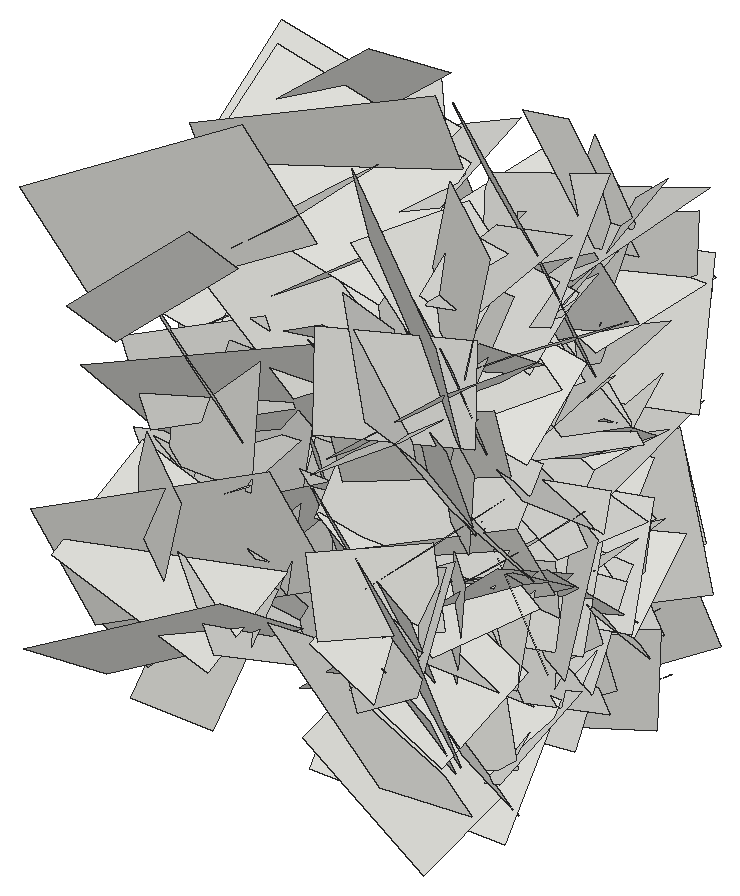
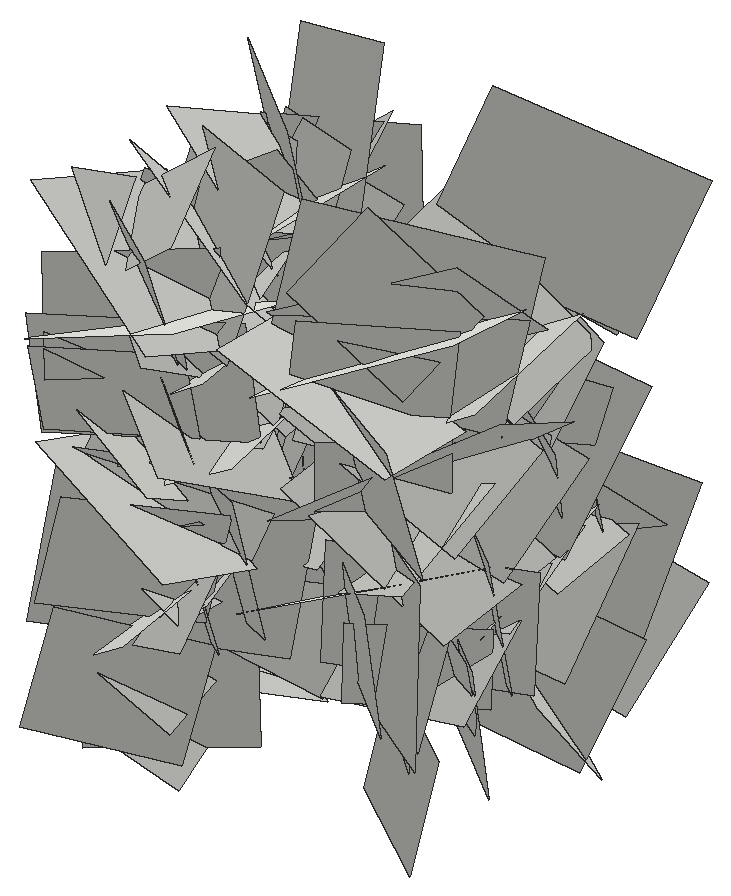
# SketchUp Ruby script. Lengths in inches.
U = 1.inch
M = Sketchup.active_model
def pt(a) = Geom::Point3d.new(a.map { |v| v * U })
def face(e, loops, mat)
  f = e.add_face(loops[0].map { |a| pt(a) })
  loops[1..].each { |l| e.add_face(l.map { |a| pt(a) }).erase! }
  f.material = f.back_material = mat if mat
  f
end
# faces: each face lists its corners as indices into pts; further lists are holes
def faces(e, pts, list, mat = nil) = list.each { |f| face(e, (f[0].is_a?(Array) ? f : [f]).map { |l| l.map { |i| pts[i] } }, mat) }
# xy, xz, yz: faces in a plane at the given z, y or x. An outline is a flat list of corners, or four numbers for a rectangle; further outlines are holes
def ring(l) = l.size == 4 ? [[l[0], l[1]], [l[2], l[1]], [l[2], l[3]], [l[0], l[3]]] : l.each_slice(2).to_a
def flat(e, list, mat, &to3) = list.each { |f| face(e, (f[0].is_a?(Array) ? f : [f]).map { |l| ring(l).map { |u, v| to3.(u, v) } }, mat) }
def xy(e, z, list, mat = nil) = flat(e, list, mat) { |x, y| [x, y, z] }
def xz(e, y, list, mat = nil) = flat(e, list, mat) { |x, z| [x, y, z] }
def yz(e, x, list, mat = nil) = flat(e, list, mat) { |y, z| [x, y, z] }
def lines(e, pts, list) = list.each { |a, b| e.add_line(pt(pts[a]), pt(pts[b])) }
# prism: a flat outline (further loops are holes) pulled along v
def prism(e, loops, v, mat = nil)
  f = face(e, loops, mat); d = Geom::Vector3d.new(v.map { |x| x * U })
  f.pushpull(f.normal.samedirection?(d) ? d.length : -d.length)
end
def box(e, o, s, mat = nil) = prism(e, [[o, [o[0] + s[0], o[1], o[2]], [o[0] + s[0], o[1] + s[1], o[2]], [o[0], o[1] + s[1], o[2]]]], [0, 0, s[2]], mat)
def at(x, y, z, deg = 0) = Geom::Transformation.translation(pt([x, y, z])) * Geom::Transformation.rotation(ORIGIN, Z_AXIS, deg.degrees)
def axes(o, x, y, z) = Geom::Transformation.new([*x, 0, *y, 0, *z, 0, *pt(o).to_a, 1])
def part(name) = M.definitions.add(name)
# library, detail: a bought-in or finely detailed component or shape, given as its bounding box
def library(name, o, s) = part(name).tap { |d| box(d.entities, o, s) }
def detail(e, o, s) = box(e.add_group.entities, o, s)
def put(e, d, t, mat = nil) = e.add_instance(d, t).tap { |i| i.material = mat if mat }
def group(e, t, mat = nil) = e.add_group.tap { |g| g.transformation = t; g.material = mat if mat }.entities
root = M.entities
c1 = part("Component\#6")
p = [[0.01,0,0],[0,3.24,4.54],[4.32,3.24,4.54],[4.33,0,0]]
faces(c1.entities,p,[[0,1,2,3]])
put(root,c1,axes([14.53,152.65,32.7],[-0.31384,1.21799,0.62272],[-0.13011,0.61092,-1.25326],[1.44417,0.31973,0.02242]))
put(root,c1,axes([14.53,149.65,34.23],[-0.2234,-0.54463,1.08834],[-0.02633,1.10624,0.54877],[1.28976,-0.07175,0.19972]))
put(root,c1,axes([18.5,152.7,33.94],[0.15183,0.13661,-0.74127],[-0.04087,-0.75222,-0.14607],[-0.79793,0.06452,-0.13357]))
put(root,c1,axes([18.5,158.73,27.09],[0.13155,-0.14233,-0.74779],[0.00006,-0.75766,0.14422],[-0.80689,-0.02326,-0.12191]))
put(root,c1,axes([14.53,158.66,27.8],[0.19419,0.10037,-0.91545],[-0.10975,-0.92523,-0.12216],[0.97001,-0.12478,0.16945]))
put(root,c1,axes([18.5,156.65,23.33],[-0.01341,0.01203,0.69899],[0.10657,0.69187,-0.01009],[-0.73333,0.10033,-0.01425]))
put(root,c1,axes([14.53,154.96,37.56],[-0.27688,1.1515,0.31839],[0.11464,0.34737,-1.16756],[1.26119,0.22122,0.17603]))
put(root,c1,axes([14.53,152.42,20.54],[-0.05004,-0.6691,0.77955],[0.05919,0.77755,0.67076],[1.08735,-0.07312,-0.00064]))
put(root,c1,axes([18.5,161,38.46],[0.19651,-0.13504,-0.81499],[0.03185,-0.8336,0.14496],[-0.87508,-0.06067,-0.17773]))
put(root,c1,axes([14.53,159.15,23.91],[0.14407,0.13595,-0.90237],[-0.02833,-0.91134,-0.14133],[0.9669,-0.04696,0.13032]))
put(root,c1,axes([14.53,151.25,34.8],[0.16779,0.3958,-0.75565],[0.05631,-0.77163,-0.39305],[0.90246,-0.02545,0.16502]))
put(root,c1,axes([18.5,158.03,24.73],[0.19324,-0.05037,0.89121],[0.15909,0.89838,0.02008],[-0.93272,0.1428,0.18806]))
put(root,c1,axes([14.53,154.4,23.625],[-0.0407,-0.65785,-0.83395],[0.03781,-0.83482,0.65689],[1.12528,0.00426,-0.05223]))
put(root,c1,axes([18.5,157.59,40.82],[0.16311,0.68993,-0.43022],[0.09586,-0.44966,-0.68876],[-0.85651,0.08106,-0.15901]))
put(root,c1,axes([14.53,154.59,24.16],[-0.1724,0.15274,1.09758],[0.17194,1.10067,-0.12914],[1.16199,-0.14021,0.18195]))
put(root,c1,axes([14.53,152.14,28.92],[0.00837,0.82237,-0.50147],[0.16225,-0.49618,-0.8113],[1.00803,0.07304,0.13474]))
put(root,c1,axes([18.5,149.08,38.35],[-0.0057,0.54335,-0.52891],[0.23788,-0.50408,-0.52014],[-0.76776,-0.16022,-0.15723]))
put(root,c1,axes([18.5,157.4,31.875],[0.05779,-0.51798,-0.36432],[0.0587,-0.36037,0.52065],[-0.6687,-0.0764,0.01422]))
put(root,c1,axes([14.53,156.45,32.24],[0.14884,0.843,-0.57449],[-0.06248,-0.57223,-0.85409],[1.07954,-0.14935,0.02978]))
put(root,c1,axes([18.5,160.09,33.87],[0.13785,-0.16653,-0.67513],[0.04892,-0.68326,0.17743],[-0.73546,-0.07666,-0.11474]))
put(root,c1,axes([14.53,156.02,28.65],[-0.0619,-0.85924,0.62732],[0.17366,0.61351,0.85557],[1.11425,-0.14335,-0.09849]))
put(root,c1,axes([18.5,147.9,27.03],[0.12769,0.03013,0.63893],[0.01482,0.64988,-0.03329],[-0.67785,0.01989,0.11963]))
put(root,c1,axes([14.53,156.69,29.48],[-0.02364,1.01192,0.31394],[0.16386,0.31376,-1.00035],[1.11105,-0.02474,0.15421]))
put(root,c1,axes([14.53,161.68,35.57],[-0.09547,-0.29138,-1.10436],[0.14499,-1.10257,0.27976],[1.20197,0.10985,-0.12146]))
put(root,c1,axes([14.53,147.58,26.68],[0.22766,0.71104,0.67114],[-0.02672,0.69094,-0.72395],[1.03608,-0.13842,-0.16614]))
put(root,c1,axes([14.53,153.43,27.14],[0.15407,-0.97446,-0.01303],[0.08051,-0.00181,0.98239],[1.02988,0.14592,-0.07485]))
put(root,c1,axes([14.53,158.93,27.77],[-0.0679,-1.16178,0.21088],[0.08573,0.20637,1.16154],[1.24867,-0.07734,-0.06828]))
put(root,c1,axes([14.53,160.05,30.35],[-0.12426,0.20575,-1.35522],[-0.11745,-1.35714,-0.19646],[1.44825,-0.0924,-0.13221]))
put(root,c1,axes([14.53,157.84,26.69],[0.16666,-0.37984,-0.88441],[0.10341,-0.88523,0.39754],[1.01503,0.15255,0.10471]))
put(root,c1,axes([14.53,153.58,31.99],[0.17505,-0.32324,-0.90395],[0.10086,-0.9072,0.34179],[1.0126,0.14624,0.12223]))
put(root,c1,axes([14.53,151.45,29.33],[0.11063,1.17252,-0.59491],[-0.28501,-0.56514,-1.16101],[1.36425,-0.21315,-0.19431]))
put(root,c1,axes([14.53,155.57,33.875],[0.13701,-1.11756,0.11199],[-0.07264,0.10468,1.12363],[1.18833,0.13525,0.05577]))
put(root,c1,axes([14.53,156.79,29.67],[0.01777,-0.29003,-1.18393],[-0.05362,-1.18318,0.28913],[1.29096,-0.04516,0.0283]))
put(root,c1,axes([14.53,158.37,30.5],[0.12568,-1.12455,0.31778],[-0.06348,0.31314,1.13049],[1.23707,0.13032,0.02572]))
put(root,c1,axes([14.53,152.25,36.24],[-0.0137,1.21221,-0.26433],[0.01965,-0.26413,-1.21218],[1.31499,0.01657,0.01536]))
put(root,c1,axes([14.53,150.2,21.48],[0.03659,-0.96074,0.6365],[0.08804,0.6372,0.9573],[1.21843,-0.01719,-0.08829]))
put(root,c1,axes([14.53,149.67,23.37],[-0.09539,-0.59855,1.14231],[0.08783,1.14003,0.60389],[1.36418,-0.11525,0.041]))
put(root,c1,axes([14.53,153.92,36.42],[0.14295,0.82362,0.79821],[0.11339,0.79118,-0.83443],[1.21047,-0.17138,-0.0161]))
put(root,c1,axes([14.53,156.14,33.68],[0.06217,-0.55405,1.15944],[0.03014,1.16092,0.55332],[1.36179,-0.0004,-0.06518]))
put(root,c1,axes([14.53,157.5625,26.25],[0.15158,-0.38022,-1.22414],[-0.0526,-1.23246,0.37701],[1.35773,-0.0053,0.15127]))
put(root,c1,axes([14.53,161.74,34.71],[0.1652,-1.10091,-0.16395],[0.26327,-0.12698,1.08875],[1.15009,0.1872,-0.22568]))
put(root,c1,axes([14.53,153.73,28.3],[-0.01858,0.99462,-0.84655],[0.29457,-0.8244,-0.97435],[1.35277,0.19318,0.20054]))
put(root,c1,axes([14.53,153.125,28.17],[-0.03085,-0.9293,0.97672],[0.26234,0.95667,0.91759],[1.40479,-0.19906,-0.14991]))
put(root,c1,axes([14.53,153.14,23.91],[0.18,-1.08552,0.79109],[0.08355,0.80406,1.08641],[1.42134,0.0902,-0.16405]))
put(root,c1,axes([28.31,153.14,23.91],[-0.18,-1.08552,0.79109],[-0.08355,0.80406,1.08641],[-1.42134,0.0902,-0.16405]))
put(root,c1,axes([28.31,153.125,28.17],[0.03085,-0.9293,0.97672],[-0.26234,0.95667,0.91759],[-1.40479,-0.19906,-0.14991]))
put(root,c1,axes([28.31,153.73,28.3],[0.01858,0.99462,-0.84655],[-0.29457,-0.8244,-0.97435],[-1.35277,0.19318,0.20054]))
put(root,c1,axes([28.31,161.74,34.71],[-0.1652,-1.10091,-0.16395],[-0.26327,-0.12698,1.08875],[-1.15009,0.1872,-0.22568]))
put(root,c1,axes([28.31,157.5625,26.25],[-0.15158,-0.38022,-1.22414],[0.0526,-1.23246,0.37701],[-1.35773,-0.0053,0.15127]))
put(root,c1,axes([28.31,156.14,33.68],[-0.06217,-0.55405,1.15944],[-0.03014,1.16092,0.55332],[-1.36179,-0.0004,-0.06518]))
put(root,c1,axes([28.31,153.92,36.42],[-0.14295,0.82362,0.79821],[-0.11339,0.79118,-0.83443],[-1.21047,-0.17138,-0.0161]))
put(root,c1,axes([28.31,149.67,23.37],[0.09539,-0.59855,1.14231],[-0.08783,1.14003,0.60389],[-1.36418,-0.11525,0.041]))
put(root,c1,axes([28.31,150.2,21.48],[-0.03659,-0.96074,0.6365],[-0.08804,0.6372,0.9573],[-1.21843,-0.01719,-0.08829]))
put(root,c1,axes([28.31,152.25,36.24],[0.0137,1.21221,-0.26433],[-0.01965,-0.26413,-1.21218],[-1.31499,0.01657,0.01536]))
put(root,c1,axes([28.31,158.37,30.5],[-0.12568,-1.12455,0.31778],[0.06348,0.31314,1.13049],[-1.23707,0.13032,0.02572]))
put(root,c1,axes([28.31,156.79,29.67],[-0.01777,-0.29003,-1.18393],[0.05362,-1.18318,0.28913],[-1.29096,-0.04516,0.0283]))
put(root,c1,axes([28.31,155.57,33.875],[-0.13701,-1.11756,0.11199],[0.07264,0.10468,1.12363],[-1.18833,0.13525,0.05577]))
put(root,c1,axes([28.31,151.45,29.33],[-0.11063,1.17252,-0.59491],[0.28501,-0.56514,-1.16101],[-1.36425,-0.21315,-0.19431]))
put(root,c1,axes([28.31,153.58,31.99],[-0.17505,-0.32324,-0.90395],[-0.10086,-0.9072,0.34179],[-1.0126,0.14624,0.12223]))
put(root,c1,axes([28.31,157.84,26.69],[-0.16666,-0.37984,-0.88441],[-0.10341,-0.88523,0.39754],[-1.01503,0.15255,0.10471]))
put(root,c1,axes([28.31,160.05,30.35],[0.12426,0.20575,-1.35522],[0.11745,-1.35714,-0.19646],[-1.44825,-0.0924,-0.13221]))
put(root,c1,axes([28.31,158.93,27.77],[0.0679,-1.16178,0.21088],[-0.08573,0.20637,1.16154],[-1.24867,-0.07734,-0.06828]))
put(root,c1,axes([28.31,153.43,27.14],[-0.15407,-0.97446,-0.01303],[-0.08051,-0.00181,0.98239],[-1.02988,0.14592,-0.07485]))
put(root,c1,axes([28.31,147.58,26.68],[-0.22766,0.71104,0.67114],[0.02672,0.69094,-0.72395],[-1.03608,-0.13842,-0.16614]))
put(root,c1,axes([28.31,161.68,35.57],[0.09547,-0.29138,-1.10436],[-0.14499,-1.10257,0.27976],[-1.20197,0.10985,-0.12146]))
put(root,c1,axes([28.31,156.69,29.48],[0.02364,1.01192,0.31394],[-0.16386,0.31376,-1.00035],[-1.11105,-0.02474,0.15421]))
put(root,c1,axes([24.34,147.9,27.03],[-0.12769,0.03013,0.63893],[-0.01482,0.64988,-0.03329],[0.67785,0.01989,0.11963]))
put(root,c1,axes([28.31,156.02,28.65],[0.0619,-0.85924,0.62732],[-0.17366,0.61351,0.85557],[-1.11425,-0.14335,-0.09849]))
put(root,c1,axes([24.34,160.09,33.87],[-0.13785,-0.16653,-0.67513],[-0.04892,-0.68326,0.17743],[0.73546,-0.07666,-0.11474]))
put(root,c1,axes([28.31,156.45,32.24],[-0.14884,0.843,-0.57449],[0.06248,-0.57223,-0.85409],[-1.07954,-0.14935,0.02978]))
put(root,c1,axes([24.34,157.4,31.875],[-0.05779,-0.51798,-0.36432],[-0.0587,-0.36037,0.52065],[0.6687,-0.0764,0.01422]))
put(root,c1,axes([24.34,149.08,38.35],[0.0057,0.54335,-0.52891],[-0.23788,-0.50408,-0.52014],[0.76776,-0.16022,-0.15723]))
put(root,c1,axes([28.31,152.14,28.92],[-0.00837,0.82237,-0.50147],[-0.16225,-0.49618,-0.8113],[-1.00803,0.07304,0.13474]))
put(root,c1,axes([28.31,154.59,24.16],[0.1724,0.15274,1.09758],[-0.17194,1.10067,-0.12914],[-1.16199,-0.14021,0.18195]))
put(root,c1,axes([24.34,157.59,40.82],[-0.16311,0.68993,-0.43022],[-0.09586,-0.44966,-0.68876],[0.85651,0.08106,-0.15901]))
put(root,c1,axes([28.31,154.4,23.625],[0.0407,-0.65785,-0.83395],[-0.03781,-0.83482,0.65689],[-1.12528,0.00426,-0.05223]))
put(root,c1,axes([24.34,158.03,24.73],[-0.19324,-0.05037,0.89121],[-0.15909,0.89838,0.02008],[0.93272,0.1428,0.18806]))
put(root,c1,axes([28.31,151.25,34.8],[-0.16779,0.3958,-0.75565],[-0.05631,-0.77163,-0.39305],[-0.90246,-0.02545,0.16502]))
put(root,c1,axes([28.31,159.15,23.91],[-0.14407,0.13595,-0.90237],[0.02833,-0.91134,-0.14133],[-0.9669,-0.04696,0.13032]))
put(root,c1,axes([24.34,161,38.46],[-0.19651,-0.13504,-0.81499],[-0.03185,-0.8336,0.14496],[0.87508,-0.06067,-0.17773]))
put(root,c1,axes([28.31,152.42,20.54],[0.05004,-0.6691,0.77955],[-0.05919,0.77755,0.67076],[-1.08735,-0.07312,-0.00064]))
put(root,c1,axes([28.31,154.96,37.56],[0.27688,1.1515,0.31839],[-0.11464,0.34737,-1.16756],[-1.26119,0.22122,0.17603]))
put(root,c1,axes([24.34,156.65,23.33],[0.01341,0.01203,0.69899],[-0.10657,0.69187,-0.01009],[0.73333,0.10033,-0.01425]))
put(root,c1,axes([28.31,158.66,27.8],[-0.19419,0.10037,-0.91545],[0.10975,-0.92523,-0.12216],[-0.97001,-0.12478,0.16945]))
put(root,c1,axes([24.34,158.73,27.09],[-0.13155,-0.14233,-0.74779],[-0.00006,-0.75766,0.14422],[0.80689,-0.02326,-0.12191]))
put(root,c1,axes([24.34,152.7,33.94],[-0.15183,0.13661,-0.74127],[0.04087,-0.75222,-0.14607],[0.79793,0.06452,-0.13357]))
put(root,c1,axes([28.31,149.65,34.23],[0.2234,-0.54463,1.08834],[0.02633,1.10624,0.54877],[-1.28976,-0.07175,0.19972]))
put(root,c1,axes([28.31,152.65,32.7],[0.31384,1.21799,0.62272],[0.13011,0.61092,-1.25326],[-1.44417,0.31973,0.02242]))
put(root,c1,axes([24.34,153.52,29.46],[-0.08102,0.00764,-0.81457],[-0.10707,-0.81193,0.00187],[0.85682,-0.10074,-0.07679]))
put(root,c1,axes([24.34,158.01,30.39],[0.08038,-0.60995,0.00551],[-0.02253,0.00291,0.6143],[0.64618,0.07598,0.02073]))
put(root,c1,axes([24.34,151.89,27.92],[0.07457,-0.37507,-0.49968],[-0.035,-0.50437,0.37394],[0.66135,0.0156,0.07613]))
put(root,c1,axes([28.31,158.65,23.12],[0.03,-0.65446,0.65644],[-0.11713,0.64968,0.65248],[-0.97555,-0.09812,-0.05816]))
put(root,c1,axes([24.34,150.81,32.67],[-0.03105,-0.70657,0.01303],[0.00041,0.01303,0.70717],[0.74909,-0.02929,0.00015]))
put(root,c1,axes([28.31,155.99,38.05],[-0.0315,0.52335,-0.79271],[0.01447,-0.79278,-0.52391],[-1.00678,-0.02777,0.01727]))
put(root,c1,axes([24.34,155.3,36.05],[-0.02231,-0.46484,-0.62566],[-0.10069,-0.6197,0.4636],[0.82005,-0.08874,0.0399]))
put(root,c1,axes([28.31,160.9375,37.33],[-0.13153,0.12633,-0.90974],[0.10231,-0.91113,-0.13969],[-0.96819,-0.11344,0.10882]))
put(root,c1,axes([28.31,153.79,24.7],[0.00565,-0.43188,0.90191],[0.04751,0.90112,0.43124],[-1.05892,0.03812,0.02416]))
put(root,c1,axes([28.31,152.27,30.34],[-0.04267,0.47891,-0.74389],[-0.05776,-0.74459,-0.47642],[-0.93603,0.02411,0.06331]))
put(root,c1,axes([28.31,150.92,33.45],[0.01124,-0.40239,0.85237],[-0.02564,0.85203,0.40253],[-0.99881,-0.0264,-0.00074]))
put(root,c1,axes([24.34,153.82,25.23],[0.04726,-0.11023,0.59197],[0.093,0.58845,0.10297],[0.63147,-0.07841,-0.05947]))
put(root,c1,axes([24.34,149.71,29.1],[0.04042,0.22115,-0.567],[0.10046,-0.56334,-0.21335],[0.63725,0.07479,0.0696]))
put(root,c1,axes([28.31,154.45,36.57],[-0.07713,0.81709,0.22722],[-0.03645,0.22503,-0.82021],[-0.89825,-0.07929,0.01378]))
put(root,c1,axes([24.34,158.75,26.14],[0.12859,0.59437,-0.23179],[-0.06253,-0.22448,-0.60651],[0.67335,-0.13435,-0.01206]))
put(root,c1,axes([28.31,156.72,22.08],[0.00521,-0.94479,0.50901],[0.17637,0.50353,0.93301],[-1.12382,0.07464,0.14878]))
put(root,c1,axes([24.34,156.34,37.48],[-0.20366,-0.78098,-0.33642],[0.07649,-0.35863,0.79133],[0.89812,-0.14656,-0.14368]))
put(root,c1,axes([28.31,150.56,37.37],[-0.01495,0.72639,-0.4873],[-0.06872,-0.48689,-0.7239],[-0.92463,0.02444,0.06168]))
put(root,c1,axes([24.34,156.49,28.09],[0.01227,0.36562,0.53928],[0.0952,0.53332,-0.36351],[0.68404,-0.08079,0.04092]))
put(root,c1,axes([28.31,150.4,30.92],[-0.04252,-0.27759,0.76161],[-0.13298,0.75548,0.26875],[-0.84891,-0.10444,-0.08025]))
put(root,c1,axes([28.31,152.31,24.83],[-0.14132,0.38772,0.61473],[-0.11706,0.60692,-0.40674],[-0.76145,-0.16526,-0.05156]))
put(root,c1,axes([24.34,150.69,21.46],[-0.08617,-0.06424,0.73191],[0.1147,0.7273,0.07585],[0.77031,-0.11548,0.07058]))
put(root,c1,axes([24.34,149.63,26.39],[-0.05575,0.3601,-0.58557],[0.15834,-0.56726,-0.36226],[0.71127,0.15451,0.03475]))
put(root,c1,axes([24.34,153.92,21.15],[-0.0271,-0.2919,0.8704],[-0.20523,0.85287,0.28034],[0.95124,0.17569,0.08528]))
put(root,c1,axes([24.34,159.1875,20.3125],[-0.01409,-0.35632,0.80543],[-0.16766,0.79339,0.34838],[0.91839,0.13938,0.07596]))
put(root,c1,axes([28.31,157.73,31.39],[0.13129,-0.92283,0.37392],[-0.04334,0.37177,0.93107],[-1.05456,-0.13017,0.00829]))
put(root,c1,axes([24.34,147.16,24.1],[-0.03025,0.92414,0.23442],[-0.23339,0.2218,-0.90118],[0.98329,0.08108,-0.20669]))
put(root,c1,axes([24.34,159.76,21.63],[0.09665,-0.666,0.12875],[-0.03078,0.12595,0.67212],[0.71837,0.095,0.01147]))
put(root,c1,axes([28.31,154.61,36.92],[0.07328,1.03426,0.55463],[0.26621,0.52968,-1.01904],[-1.21518,0.17841,-0.1898]))
put(root,c1,axes([24.34,160.84,30.26],[0.09118,-0.56201,-0.30691],[0.0596,-0.30185,0.56849],[0.67615,0.1024,-0.00872]))
put(root,c1,axes([24.34,156.05,22.34],[0.04217,-0.56806,-0.37659],[0.07293,-0.37196,0.56834],[0.71876,0.07107,-0.03557]))
put(root,c1,axes([28.31,158.82,28.52],[0.0834,-0.34729,-0.88838],[-0.00654,-0.89156,0.34799],[-1.01106,-0.02288,-0.07553]))
put(root,c1,axes([28.31,151.53,22],[0.08087,0.78957,0.40941],[-0.10212,0.41583,-0.78401],[-0.93722,0.02282,0.12075]))
put(root,c1,axes([28.31,152.86,25.21],[-0.07237,-0.84668,-0.40971],[0.16913,-0.41526,0.83156],[-0.98259,-0.00911,0.17331]))
put(root,c1,axes([28.31,150.44,37.52],[0.01758,-0.03984,-0.83316],[-0.08726,-0.82933,0.03802],[-0.87984,0.08145,-0.02042]))
put(root,c1,axes([28.31,161.57,34.4],[0.05292,-0.24359,-0.78611],[-0.1523,-0.77804,0.23197],[-0.85897,0.12294,-0.08956]))
put(root,c1,axes([24.34,154.14,39.875],[-0.07687,-0.17009,-0.90128],[-0.07958,-0.89996,0.17589],[0.96896,-0.0874,-0.05706]))
put(root,c1,axes([24.34,159.35,19.53],[0.12506,-0.65018,0.20227],[-0.00025,0.20525,0.65988],[0.72178,0.11273,-0.03482]))
put(root,c1,axes([28.31,155.63,34.51],[0.04715,-0.7148,-0.47013],[-0.06325,-0.47221,0.71232],[-0.90467,-0.00424,-0.0743]))
put(root,c1,axes([28.31,151.43,29.49],[0.01376,0.93036,0.01045],[0.09599,0.00914,-0.92605],[-0.98156,0.01394,-0.09041]))
put(root,c1,axes([28.31,156.02,27.27],[-0.01737,0.78195,0.05447],[-0.0729,0.05284,-0.77921],[-0.82768,-0.02106,0.06749]))
put(root,c1,axes([24.34,152.23,36.27],[0.17612,0.33723,0.58016],[-0.03508,0.60107,-0.33991],[0.71045,-0.05392,-0.16061]))
put(root,c1,axes([24.34,152.86,32.22],[-0.07765,-0.95123,0.12327],[-0.10469,0.13045,0.94796],[1.01133,-0.05954,0.1076]))
put(root,c1,axes([28.31,160.42,26.72],[0.04031,-0.6417,-0.5437],[-0.04231,-0.54502,0.64047],[-0.89052,-0.00315,-0.05504]))
put(root,c1,axes([24.34,153.18,27.99],[-0.08911,-1.01671,-0.11332],[-0.1646,-0.0997,1.00972],[1.07181,-0.09984,0.14565]))
